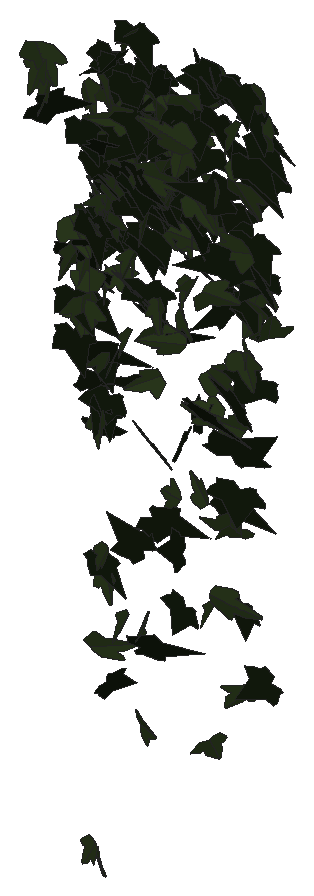
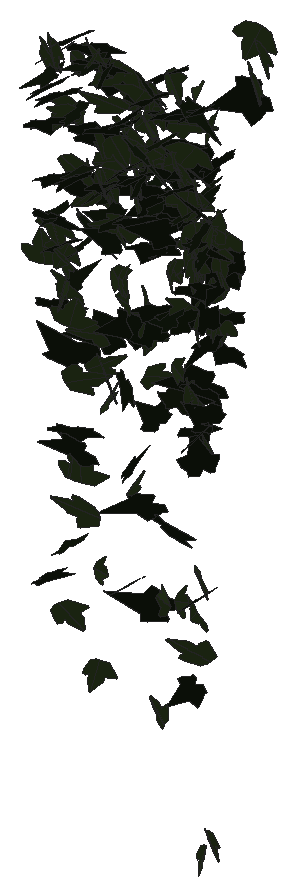
# SketchUp Ruby script. Lengths in millimetres.
U = 1.mm
M = Sketchup.active_model
def pt(a) = Geom::Point3d.new(a.map { |v| v * U })
def face(e, loops, mat)
  f = e.add_face(loops[0].map { |a| pt(a) })
  loops[1..].each { |l| e.add_face(l.map { |a| pt(a) }).erase! }
  f.material = f.back_material = mat if mat
  f
end
# faces: each face lists its corners as indices into pts; further lists are holes
def faces(e, pts, list, mat = nil) = list.each { |f| face(e, (f[0].is_a?(Array) ? f : [f]).map { |l| l.map { |i| pts[i] } }, mat) }
# xy, xz, yz: faces in a plane at the given z, y or x. An outline is a flat list of corners, or four numbers for a rectangle; further outlines are holes
def ring(l) = l.size == 4 ? [[l[0], l[1]], [l[2], l[1]], [l[2], l[3]], [l[0], l[3]]] : l.each_slice(2).to_a
def flat(e, list, mat, &to3) = list.each { |f| face(e, (f[0].is_a?(Array) ? f : [f]).map { |l| ring(l).map { |u, v| to3.(u, v) } }, mat) }
def xy(e, z, list, mat = nil) = flat(e, list, mat) { |x, y| [x, y, z] }
def xz(e, y, list, mat = nil) = flat(e, list, mat) { |x, z| [x, y, z] }
def yz(e, x, list, mat = nil) = flat(e, list, mat) { |y, z| [x, y, z] }
def lines(e, pts, list) = list.each { |a, b| e.add_line(pt(pts[a]), pt(pts[b])) }
# prism: a flat outline (further loops are holes) pulled along v
def prism(e, loops, v, mat = nil)
  f = face(e, loops, mat); d = Geom::Vector3d.new(v.map { |x| x * U })
  f.pushpull(f.normal.samedirection?(d) ? d.length : -d.length)
end
def box(e, o, s, mat = nil) = prism(e, [[o, [o[0] + s[0], o[1], o[2]], [o[0] + s[0], o[1] + s[1], o[2]], [o[0], o[1] + s[1], o[2]]]], [0, 0, s[2]], mat)
def at(x, y, z, deg = 0) = Geom::Transformation.translation(pt([x, y, z])) * Geom::Transformation.rotation(ORIGIN, Z_AXIS, deg.degrees)
def axes(o, x, y, z) = Geom::Transformation.new([*x, 0, *y, 0, *z, 0, *pt(o).to_a, 1])
def part(name) = M.definitions.add(name)
# library, detail: a bought-in or finely detailed component or shape, given as its bounding box
def library(name, o, s) = part(name).tap { |d| box(d.entities, o, s) }
def detail(e, o, s) = box(e.add_group.entities, o, s)
def put(e, d, t, mat = nil) = e.add_instance(d, t).tap { |i| i.material = mat if mat }
def group(e, t, mat = nil) = e.add_group.tap { |g| g.transformation = t; g.material = mat if mat }.entities
root = M.entities
M.materials.add("efeu1").color = [18, 25, 13]
M.materials.add("efeu2").color = [43, 57, 29]
c1 = part("ivyleaf_10")
p = [[0,12.8,-0.8],[-1.5,51.3,-10.9],[-4.9,51,-11.6],[-13.6,26.5,-7.3],[-13.2,15.9,-4.6],[-21.1,19.3,-7.2],
  [-29.5,16.3,-8.3],[-29.2,8.3,-6.2],[-19.7,-9.8,0.5],[-7.6,-13,4],[1,-12.2,5.8],[-0.4,51.1,-11.1],
  [-1.5,51.1,-10.9],[1,-12.4,5.9],[16.9,-12.4,3.5],[35.1,9.1,-5.1],[35,12.9,-6.1],[20.5,16.4,-4.9],
  [15.8,15,-3.8],[15.3,27.6,-7.1],[12.8,31.3,-7.8]]
faces(c1.entities,p,[[0,1,2,3,4,5,6,7,8,9,10],[11,12,0,13,14,15,16,17,18,19,20]],"efeu2")
c2 = part("ivyleaf_9")
p = [[39.1,54.8,31.7],[34.5,51.8,30.2],[-5.3,25.2,17.3],[-17.9,28.3,20.9],[-21.6,21.7,17],[-20.2,4.3,5.3],
  [-22.9,-0.3,2.5],[-17.1,-4,-0.6],[-2,-2.1,-1.2],[-0.7,-15.4,-10.1],[16.6,-22.3,-16.7],[21.1,-15.1,-12.5],
  [32.7,-10.7,-11],[46.1,-1.8,-6.6],[30.8,11.2,3.8]]
faces(c2.entities,p,[[0,1,2,3,4,5,6,7,8,9,10,11,12,13,14]],"efeu1")
put(root,c1,axes([827.3,914.8,1269.9],[-0.03685,-0.91844,-0.1147],[0.01699,0.11429,-0.91888],[1.12908,-0.0317,0.01008]))
put(root,c2,axes([810.5,984.3,656.7],[0.43148,-0.72111,-0.27887],[-0.13514,0.26997,-0.75581],[1.46526,0.23725,0.01241]))
put(root,c1,axes([816.5,990.8,1433.1],[0.58304,-0.45427,0.49056],[0.46498,-0.31033,-0.65866],[0.67017,0.61052,0.03022]))
put(root,c2,axes([814.6,955.2,977],[-0.06259,-0.1793,0.84576],[0.93108,0.38869,0.1287],[-0.49559,0.7529,0.13498]))
put(root,c2,axes([815,917.2,1162.1],[-0.08072,-0.79037,-0.52122],[0.18121,0.50735,-0.7882],[1.14074,-0.13652,0.08832]))
put(root,c1,axes([825.2,950.5,1338.1],[-0.84236,0.60608,-0.07259],[0.08412,-0.03146,-0.91848],[-0.73994,-0.69356,-0.02178]))
put(root,c1,axes([826.2,828.6,1581.8],[0.96241,-0.8078,0.0551],[0.0642,-0.02561,-1.12892],[0.98571,0.79037,0.01973]))
put(root,c2,axes([814.5,970.2,1305.8],[0.80675,-0.56254,-0.10977],[-0.09704,0.07591,-0.86815],[0.69247,0.66601,0.00623]))
put(root,c1,axes([832.2,935.6,168.4],[0.72355,-0.48205,-0.26083],[-0.2237,0.18766,-0.76374],[0.63014,0.62013,0.02837]))
put(root,c1,axes([830.4,897.2,1252.3],[0.06343,-0.81421,0.59742],[0.10119,-0.59274,-0.81506],[1.22788,0.09091,0.03631]))
put(root,c1,axes([828.7,808.1,1627.5],[1.11625,-0.68472,-0.01362],[-0.00812,0.01384,-1.14278],[0.83549,0.91496,0.00709]))
put(root,c1,axes([830.8,966.8,680.9],[0.75004,-0.66968,0.01112],[0.01074,-0.00958,-0.77704],[1.27467,0.39414,0]))
put(root,c2,axes([819.4,971.6,896.5],[1.00535,0.15537,0.12513],[-0.16841,0.06015,0.83438],[0.17571,-0.83133,0.08376]))
put(root,c2,axes([829.7,901.7,1243.4],[0.57474,0.86858,0.16422],[0.0941,0.14499,-0.98811],[-1.07432,0.47737,0.00131]))
put(root,c1,axes([830.9,912.7,1152.6],[-0.32089,-0.95674,0.05571],[0.17709,-0.09687,-0.97836],[1.15571,-0.2508,0.16538]))
put(root,c2,axes([814.6,967.4,1167.5],[-0.16658,-0.25139,0.83172],[0.71275,-0.64976,-0.10048],[0.78464,0.53686,0.26785]))
put(root,c2,axes([832.3,992.7,1245.9],[-0.67217,-0.65377,0.02912],[-0.00914,-0.03177,-0.85484],[0.79834,-0.55081,0.01473]))
put(root,c2,axes([819.6,907.6,1097],[-0.57889,-0.38228,-0.72656],[0.81391,0.30957,-0.59856],[0.58377,-0.81069,0.11404]))
put(root,c1,axes([821.6,984.9,1164.7],[0.39568,-0.50354,0.60933],[0.54283,-0.42808,-0.59059],[0.79708,0.5415,0.09973]))
put(root,c1,axes([815.7,989.8,623.1],[0.90908,-0.34629,0.5412],[0.8315,-0.3194,-0.58998],[0.89659,0.64733,-0.00159]))
put(root,c2,axes([822.2,923.6,1464.6],[0.22176,-0.83835,-0.36779],[-0.07301,0.36329,-0.85766],[1.11449,0.19061,0.017]))
put(root,c2,axes([824.6,945.8,1125.8],[0.31626,-0.49164,-0.71685],[-0.23548,0.69682,-0.5477],[1.03401,0.30907,0.09453]))
put(root,c1,axes([837.8,947.6,142.7],[-0.61671,0.51827,0.32896],[-0.28351,0.23286,-0.72396],[-0.69317,-0.55635,0.00343]))
put(root,c1,axes([836,970.5,1276.3],[-0.1259,-0.84841,-0.28929],[0.02873,0.28853,-0.85459],[1.0932,-0.10529,-0.01086]))
put(root,c2,axes([819.1,976.3,1338.3],[0.5738,-0.73935,0.1343],[0.09718,-0.10849,-0.87622],[0.9116,0.47694,0.00887]))
put(root,c1,axes([825.9,934.6,1157.4],[-0.60213,0.51709,-0.58666],[0.41991,-0.47929,-0.71201],[-0.85669,-0.59837,0.06335]))
put(root,c2,axes([825.7,967.3,1039.2],[-0.48321,-0.46701,-0.61897],[0.59057,0.39403,-0.60704],[0.73897,-0.62027,0.0804]))
put(root,c2,axes([823.1,822.3,1544],[0.04444,0.49674,-1.00223],[0.09991,0.99889,0.49806],[1.361,-0.08955,-0.00384]))
put(root,c2,axes([856.9,952.9,1298.1],[-0.87759,0.06382,0.52703],[-0.64482,-0.00287,-0.72105],[-0.06074,-0.89174,0.04004]))
put(root,c2,axes([832,886.9,1266.4],[1.00556,0.61266,-0.081],[-0.0684,-0.06035,-1.02688],[-0.75084,0.826,-0.01494]))
put(root,c1,axes([834.4,913.6,1239.5],[0.96654,-0.59003,0.14227],[0.15072,-0.07228,-0.9877],[0.72497,0.80166,0.01566]))
put(root,c1,axes([842.5,964.1,1036.4],[-0.28327,-0.87367,0.10082],[-0.03216,-0.09732,-0.90399],[1.07247,-0.23368,-0.00048]))
put(root,c1,axes([834.3,806.9,1651.5],[-1.34063,-0.0535,-0.34198],[0.42219,-0.19472,-1.08151],[-0.00925,-1.13426,0.2018]))
put(root,c2,axes([857.3,961.7,1571.8],[-0.78827,0.67967,-0.20007],[0.06248,-0.21309,-0.79186],[-1.34698,-0.40764,0.08036]))
put(root,c1,axes([833.2,912.9,1143.7],[1.17935,0.20887,0.10557],[0.10249,0.10907,-0.98503],[-0.26649,0.96629,0.08837]))
put(root,c1,axes([839.9,919.6,1187.7],[0.35761,0.91321,-0.25171],[0.08106,0.24301,0.95905],[1.15282,-0.30037,0.01064]))
put(root,c2,axes([840.3,968.3,960.7],[-0.62655,-0.73059,-0.04307],[0.02972,0.03552,-0.89304],[0.89238,-0.51414,-0.0005]))
put(root,c2,axes([831.3,975.3,947.9],[0.11589,-0.86539,0.18702],[0.00654,-0.18752,-0.87047],[1.08013,0.09399,-0.01479]))
put(root,c2,axes([836.2,979.2,1569.9],[-0.28232,-0.79533,0.20841],[0.03217,-0.22358,-0.82392],[1.00254,-0.21679,0.08513]))
put(root,c1,axes([840,962.2,1276.7],[0.2733,-0.74511,0.25395],[0.24362,-0.2326,-0.75486],[1.47825,0.17609,0.07745]))
put(root,c1,axes([839.9,916.4,1534.1],[-0.28327,0.96823,0.01867],[-0.00068,0.01907,-0.99567],[-1.18146,-0.23216,-0.0039]))
put(root,c2,axes([828.3,936.8,1395.7],[0.91204,-0.61799,-0.26415],[-0.31818,0.20461,-0.78199],[1.23889,0.5075,-0.00638]))
put(root,c1,axes([842.3,961.9,1270.2],[0.72661,-0.63739,0.07321],[0.05935,-0.05473,-0.87234],[0.78047,0.59756,-0.00182]))
put(root,c1,axes([838.4,978.7,1497.4],[-1.42032,-0.1447,-0.26511],[0.52164,-0.02761,-0.75648],[0.24146,-0.79149,0.07486]))
put(root,c1,axes([830.1,893.2,1299.6],[1.0073,0.30023,0.54458],[0.63222,0.16817,-0.8784],[-0.41937,0.97468,-0.01619]))
put(root,c2,axes([821.9,951.3,1048.5],[0.23102,0.24737,-0.79483],[0.70014,0.70461,0.27547],[1.4212,-0.38733,-0.00651]))
put(root,c2,axes([833.9,929.7,1410.4],[0.7252,-0.56889,-0.413],[-0.12026,0.46805,-0.78661],[0.84918,0.55212,0.24129]))
put(root,c1,axes([852.8,948.7,1329.2],[-0.61781,-0.73834,0.06604],[-0.0454,-0.05455,-0.89531],[0.90323,-0.50777,0.00017]))
put(root,c1,axes([851,967.8,1040.6],[0.49501,-0.80316,-0.13013],[-0.08958,0.10868,-0.89968],[0.98859,0.41201,-0.01637]))
put(root,c1,axes([846,958.1,1297.8],[0.55063,-0.71531,0.22891],[0.2274,-0.19835,-0.77081],[1.41118,0.31107,0.03489]))
put(root,c2,axes([849.6,955.9,459.9],[-0.04951,0.15388,-0.76833],[-0.50569,0.72148,0.15349],[1.40297,0.26548,0.02821]))
put(root,c1,axes([839.5,943.2,934.3],[0.8773,-0.46081,0.55084],[0.725,-0.39799,-0.65172],[1.15869,0.59792,-0.00928]))
put(root,c2,axes([842,942.7,1283.5],[0.61468,-0.51987,-0.46856],[-0.349,0.43516,-0.60921],[1.28546,0.36674,0.05866]))
put(root,c1,axes([859.3,962.5,1394.7],[-1.26299,-0.42447,-0.01308],[0.0122,0.01425,-0.78771],[0.80813,-0.66359,-0.00855]))
put(root,c2,axes([837,982.5,1380.5],[0.52468,-0.76338,-0.1447],[-0.02366,0.14918,-0.81073],[1.47854,0.27328,0.03838]))
put(root,c2,axes([853.8,976.6,1395.7],[-1.22598,-0.10596,-0.44543],[0.8701,-0.10684,-0.63574],[0.04762,-0.77585,0.14838]))
put(root,c1,axes([835.9,952.8,519.4],[-0.59891,-0.25699,0.66664],[0.96813,0.43092,0.40624],[-0.95481,0.59812,-0.00625]))
put(root,c1,axes([856.6,947.8,1299.5],[-1.06707,0.18745,-0.06691],[0.07914,-0.01663,-0.89451],[-0.22956,-0.87705,0.00266]))
put(root,c1,axes([836.2,901.6,1312],[0.04887,-0.13965,0.93591],[1.14246,-0.12885,-0.0593],[0.166,0.92786,0.13263]))
put(root,c1,axes([853.6,989.7,1468],[1.0977,-0.51262,0.2237],[0.28993,-0.16521,-0.77135],[1.02423,0.59616,-0.0214]))
put(root,c2,axes([859.4,972,1559.8],[-0.51457,-0.76812,0.05811],[-0.03506,-0.05512,-0.81432],[1.46565,-0.271,0.00092]))
put(root,c1,axes([871.5,970.8,1479.7],[-0.08503,-0.79721,-0.08124],[0.02219,0.08071,-0.79843],[1.52495,-0.04563,0.00709]))
put(root,c1,axes([865.6,984.5,1075.2],[0.18999,-0.5844,0.42532],[0.30361,-0.40095,-0.58836],[1.34168,0.17349,0.07291]))
put(root,c1,axes([855.8,968.8,1188.3],[0.7648,0.30394,0.50272],[0.52166,0.26806,-0.69527],[-0.49146,0.75753,0.04432]))
put(root,c1,axes([879.7,938.1,1372.9],[-1.38425,-0.27933,0.11946],[-0.21646,-0.03705,-0.7791],[0.53615,-0.73614,-0.00612]))
put(root,c2,axes([855.3,912.2,1441.4],[1.05483,0.18398,0.3408],[0.39529,0.11309,-0.88305],[-0.25884,0.92245,0.04029]))
put(root,c2,axes([845.6,983.1,1171.1],[0.86645,-0.5011,0.39711],[0.55215,-0.27251,-0.67648],[1.08436,0.53916,0.02715]))
put(root,c1,axes([880.6,978.3,1624.3],[0.02986,-0.83075,0.01138],[-0.05286,-0.0119,-0.83043],[1.58035,0.0153,-0.02799]))
put(root,c2,axes([865.3,975.8,1414.6],[-0.0936,-0.78121,-0.10289],[0.02904,0.10213,-0.78271],[1.49935,-0.05075,0.00874]))
put(root,c2,axes([865.1,899.4,1315.7],[0.17257,-1.01284,0.08061],[0.00573,-0.08074,-1.02265],[1.23956,0.14138,-0.00649]))
put(root,c2,axes([867.3,978.5,1000.3],[-0.43764,-0.81464,0.01399],[0.98174,-0.35663,-0.13333],[0.15569,-0.04108,0.88008]))
put(root,c1,axes([909.1,924.2,1504.4],[0.12914,0.1045,-0.8512],[-1.35399,-0.46995,-0.1144],[-0.91143,0.71295,0.04935]))
put(root,c2,axes([867.1,985.6,1170.9],[0.8548,-0.63915,0.10465],[0.09811,-0.09167,-0.78111],[1.22873,0.45196,-0.01044]))
put(root,c2,axes([917.4,938.3,1449.3],[-0.88049,0.52655,0.39135],[-0.57502,0.25407,-0.69901],[-1.10832,-0.55013,0.05175]))
put(root,c1,axes([878.9,914,1556.1],[-0.14586,-0.23699,0.81822],[1.03542,-0.64577,-0.13608],[1.24752,0.50827,0.20861]))
put(root,c1,axes([886.5,974.1,1241.4],[0.31539,-0.57204,0.53633],[0.64416,-0.4423,-0.57633],[1.3462,0.34566,0.15012]))
put(root,c2,axes([885.5,977.5,1630.9],[0.01718,-0.81708,-0.15844],[0.01211,0.15852,-0.81709],[1.58398,0.00765,0.00797]))
put(root,c1,axes([897.2,953,1242.3],[-0.06309,-0.66304,0.38061],[0.26024,-0.37997,-0.65001],[1.43157,0.03985,0.13494]))
put(root,c1,axes([908.4,926.4,1402],[0.92414,-0.38759,-0.49857],[-0.51187,0.4421,-0.60563],[1.08744,0.53749,0.13862]))
put(root,c2,axes([927.5,941.4,732.5],[-1.28141,0.06996,-0.45742],[-0.86931,0.02883,0.67674],[0.14101,0.81346,0.01535]))
put(root,c1,axes([896.1,937.4,595.6],[0.15187,-0.35651,0.71863],[0.47374,-0.67553,-0.36277],[1.45139,0.2578,0.04321]))
put(root,c2,axes([895.4,960.8,1543.8],[-0.46175,-0.82107,0.00655],[-0.00409,-0.0062,-0.85616],[1.5627,-0.24263,-0.0003]))
put(root,c2,axes([913.7,939,1471.6],[-1.23869,-0.46626,0.07814],[-0.11513,-0.04973,-0.8006],[0.89236,-0.65363,0.00517]))
put(root,c2,axes([889.6,988.8,1501.7],[0.29657,-0.79421,0.00354],[0.00122,-0.00348,-0.80935],[1.51156,0.15583,-0.00004]))
put(root,c2,axes([896.1,962.2,1341.2],[-0.19584,-0.5204,-0.6231],[0.35633,0.59595,-0.52864],[1.50344,-0.20903,0.04412]))
put(root,c2,axes([907.6,982,1175.4],[-0.36294,-0.68504,-0.37729],[0.17046,0.36666,-0.71101],[1.47863,-0.21042,-0.01064]))
put(root,c1,axes([900,977.4,387.5],[-0.46711,0.14957,0.73666],[1.14822,-0.42307,0.2869],[0.85339,0.6511,0.0172]))
put(root,c2,axes([888.7,980.8,1323.7],[1.14436,-0.26249,0.44766],[0.80615,-0.14758,-0.65547],[0.57059,0.73495,0.02826]))
put(root,c1,axes([902.2,941.6,1434.2],[0.7684,-0.34663,0.59315],[1.03453,-0.25955,-0.52168],[0.79959,0.66893,0.10495]))
put(root,c1,axes([935.5,964.9,1028.5],[0.32745,0.19909,-0.76985],[-0.86061,-0.62341,-0.26228],[-1.24485,0.48335,-0.02118]))
put(root,c1,axes([919,959.3,1311.4],[0.60556,-0.66271,0.3683],[0.40536,-0.30521,-0.73318],[1.38485,0.37912,0.05356]))
put(root,c1,axes([928.9,933.2,578],[0.42426,-0.57055,0.53871],[-0.38516,0.49928,0.61253],[-1.4429,-0.30103,-0.00511]))
put(root,c2,axes([908.6,967.8,1367.5],[0.57251,-0.7274,0.2546],[0.16128,-0.24043,-0.78704],[1.45784,0.31225,-0.01291]))
put(root,c1,axes([933.1,967.3,1117.9],[-0.45052,-0.68474,-0.35407],[0.2004,0.33819,-0.72444],[1.45337,-0.25889,-0.00986]))
put(root,c2,axes([901.8,928.3,1408.5],[0.18764,-0.11833,-0.84681],[1.59009,0.19461,0.07008],[0.34607,-0.83002,0.13715]))
put(root,c2,axes([911.2,959.6,1359.8],[-0.36869,-0.19084,-0.77693],[1.07975,0.53085,-0.27185],[1.07354,-0.59946,0.0066]))
put(root,c2,axes([923.3,972.8,1283.1],[-0.54178,-0.66269,-0.37657],[0.30473,0.34101,-0.72116],[1.41827,-0.32642,0.0111]))
put(root,c2,axes([922.6,981.4,1570.9],[-0.13676,-0.82224,-0.03527],[0.01053,0.03492,-0.82537],[1.56629,-0.07203,0.00247]))
put(root,c2,axes([913.1,989.4,1118.9],[0.16574,-0.39271,0.67056],[0.88769,-0.51328,-0.36118],[1.18294,0.4402,0.17708]))
put(root,c2,axes([925.8,952.1,1263.5],[-0.12755,-0.65362,0.40278],[0.27795,-0.40778,-0.63743],[1.43451,0.0209,0.15932]))
put(root,c2,axes([936.9,932.8,1511],[-0.74306,-0.70933,-0.06795],[0.09515,0.05002,-0.80944],[1.35283,-0.39313,0.01961]))
put(root,c1,axes([943.9,960.8,1510.2],[0.50585,-0.7063,0.29734],[0.17142,-0.28374,-0.75451],[1.44838,0.28026,-0.01455]))
put(root,c2,axes([932.9,926.5,1386.7],[-0.25462,-0.65206,0.43289],[0.30937,-0.45274,-0.63173],[1.4571,-0.01782,0.20977]))
put(root,c2,axes([970.5,965.8,1453.9],[-0.83831,0.67683,0.17098],[-0.20886,0.13253,-0.80731],[-1.3121,-0.45353,0.01926]))
put(root,c2,axes([934.2,993.2,1407.7],[0.43695,-0.17133,-0.74563],[1.14548,-0.44014,0.28646],[-0.89889,-0.64417,0.00259]))
put(root,c2,axes([957.8,955.9,1576.1],[-1.1597,0.20437,-0.5192],[0.81946,-0.31675,-0.63001],[-0.67543,-0.73521,0.1271]))
put(root,c2,axes([945.7,991,1335.3],[-0.47467,-0.71427,-0.17879],[0.13356,0.16485,-0.75647],[1.39496,-0.25883,0.01159]))
put(root,c2,axes([952,990.8,1430.8],[-0.71976,-0.65843,0.26314],[0.01495,-0.3021,-0.74463],[1.34942,-0.34785,0.14861]))
put(root,c1,axes([940.3,961.8,1164],[0.85805,-0.40375,0.54214],[0.77291,-0.35917,-0.6052],[1.02844,0.60678,0.00251]))
put(root,c1,axes([955.7,989.8,813.5],[-0.26738,0.48935,0.50558],[0.20018,-0.49516,0.5085],[1.32407,0.17368,0.02522]))
put(root,c1,axes([952.4,929,1514.2],[-1.16331,0.48568,-0.2386],[0.31218,-0.17672,-0.77993],[-0.98141,-0.63191,0.03473]))
put(root,c2,axes([936.3,945.1,931.5],[0.36448,-0.54337,0.58497],[0.42116,-0.54187,-0.57578],[1.45998,0.29196,0.02006]))
put(root,c2,axes([949,990.4,1412.8],[-0.16291,-0.79422,-0.03519],[-0.00387,0.03561,-0.7988],[1.51304,-0.08542,-0.00583]))
put(root,c2,axes([938.6,962.5,781.4],[0.42736,-0.07733,-0.8202],[0.22047,0.84464,-0.04792],[1.55235,-0.09867,0.23261]))
put(root,c1,axes([973.2,927.5,1548.6],[-1.17822,0.40829,0.35636],[-0.5646,0.19745,-0.74158],[-0.86315,-0.68648,-0.00136]))
put(root,c1,axes([969.1,948.3,1434],[-0.38395,-0.81669,0.01919],[-0.00556,-0.01905,-0.84123],[1.55474,-0.20175,0.00173]))
put(root,c1,axes([981,957.7,1112.2],[0.061,0.08121,0.82664],[-0.68266,-0.74479,0.08707],[1.42583,-0.36007,0.00632]))
put(root,c2,axes([945,970.1,1392.2],[-0.14928,-0.31986,-0.74528],[0.83169,0.6141,-0.30955],[1.3003,-0.42951,0.11243]))
put(root,c1,axes([971.1,958.1,1375.5],[-0.06928,-0.81137,-0.1848],[0.06748,0.1833,-0.81175],[1.58231,-0.04334,0.02652]))
put(root,c2,axes([939,932.1,563.6],[0.61971,-0.01227,0.75109],[1.42891,0.0319,-0.32496],[-0.04642,0.81801,0.02394]))
put(root,c1,axes([978.5,951.2,1399.4],[0.43289,-0.63084,-0.51206],[-0.25157,0.49593,-0.66969],[1.52576,0.26075,0.03486]))
put(root,c2,axes([986.6,984.3,1502.8],[-0.62613,-0.68329,0.30857],[0.23752,0.28235,0.75831],[-1.40699,0.35174,-0.0093]))
put(root,c2,axes([975.5,947.6,1499],[-0.60959,-0.7039,0.37229],[-0.31978,-0.3325,-0.77323],[1.48138,-0.36143,-0.01372]))
put(root,c2,axes([972.3,992.9,620.2],[-0.36378,-0.61525,0.418],[-0.20113,-0.40474,-0.64406],[1.40126,-0.21782,0.01607]))
put(root,c2,axes([962.5,975.4,1427.8],[0.5553,-0.60977,-0.41938],[-0.17491,0.41745,-0.6709],[1.39759,0.29452,0.08266]))
put(root,c2,axes([966.5,961.8,1111.8],[-0.03415,0.43454,-0.70073],[-0.0144,0.70078,0.43477],[1.56919,0.01589,-0.01126]))
put(root,c1,axes([959.7,952.3,1497.6],[0.9628,-0.31608,0.5704],[0.94265,-0.28337,-0.5963],[0.80734,0.7078,0.016]))
put(root,c1,axes([969.3,945.1,1547.6],[1.36056,0.32118,0.26593],[0.42654,0.14913,-0.7826],[-0.66924,0.74802,0.04184]))
put(root,c2,axes([986.8,936.9,1514.9],[0.62803,-0.24303,-0.74984],[-1.08912,0.48517,-0.40908],[1.03169,0.66013,0.0246]))
put(root,c2,axes([991.4,904.9,1517.3],[-0.54686,0.68274,-0.50501],[-0.49269,0.43734,0.73855],[1.53931,0.38254,0.05698]))
put(root,c1,axes([991.7,985.7,1210.9],[0.02542,-0.78462,0.19416],[0.0799,-0.19325,-0.78383],[1.53625,0.02304,0.03756]))
put(root,c1,axes([957.8,919.9,1419.5],[-0.2359,-0.06632,0.87594],[1.62493,0.19901,0.13588],[-0.3933,0.86199,0.03602]))
put(root,c1,axes([981.2,985.4,1205.9],[0.11973,-0.49702,0.63173],[0.62404,-0.56268,-0.47535],[1.39676,0.294,0.15822]))
put(root,c1,axes([999.7,981,1457.1],[-0.53038,-0.71802,0.24819],[-0.11271,-0.24303,-0.76957],[1.44147,-0.28319,0.03115]))
put(root,c1,axes([980.1,972.6,1156.4],[0.3009,-0.24491,0.75063],[1.14513,-0.45833,-0.27627],[0.97306,0.61512,0.09301]))
put(root,c1,axes([989.2,981.2,1292.2],[0.59138,-0.37169,0.60793],[0.84661,-0.41692,-0.48227],[1.05941,0.54066,0.04604]))
put(root,c1,axes([980.2,969,1302.3],[-0.51325,-0.17728,-0.76835],[1.43762,0.17496,-0.30549],[0.43068,-0.79529,0.10407]))
put(root,c1,axes([1037.7,901.6,1516.2],[0.63285,0.07041,0.85628],[-1.5834,-0.20282,0.33976],[0.40819,-0.89591,-0.00962]))
put(root,c1,axes([1005.1,943.5,1469.4],[1.35775,-0.44841,0.12117],[0.17973,-0.07741,-0.84249],[0.86556,0.71947,-0.01513]))
put(root,c2,axes([1028.2,917.7,962.7],[-0.38655,0.20716,-0.8038],[-1.12391,0.54547,0.2898],[1.11019,0.62434,0.01351]))
put(root,c2,axes([1006.6,978.7,974.3],[-0.03219,0.46499,0.67833],[0.01021,-0.67839,0.46517],[1.56516,0.01399,0.01092]))
put(root,c1,axes([1026.9,967,1380.2],[1.1549,-0.18759,-0.47779],[-0.48533,0.53188,-0.5327],[0.84782,0.56001,0.3459]))
put(root,c2,axes([1030.4,977.4,1570.3],[-0.19191,-0.50517,0.65479],[0.26058,0.64033,0.5151],[-1.55224,0.16995,0.00552]))
put(root,c2,axes([1018.3,976.9,1369.4],[-0.62393,-0.70465,-0.13201],[0.07987,0.12605,-0.77703],[1.36208,-0.33017,-0.01491]))
put(root,c2,axes([1001.8,979.6,1310.1],[0.69116,-0.6093,0.3279],[0.36035,-0.26868,-0.70895],[1.26662,0.40892,0.02277]))
put(root,c1,axes([1023.6,994.8,637.9],[0.18782,-0.42814,0.5521],[0.32859,-0.52534,-0.43825],[1.28843,0.19639,0.03129]))
put(root,c2,axes([999.6,970.7,1263.2],[0.77104,-0.55256,0.4427],[0.56086,-0.33217,-0.68429],[1.22525,0.49977,0.03465]))
put(root,c2,axes([1035.3,904.4,778.8],[-0.20133,-0.06323,0.8525],[-0.75003,-0.75867,-0.10517],[1.44374,-0.40295,0.06425]))
put(root,c2,axes([1035.8,973.7,1470.2],[-0.81634,-0.65321,0.1995],[-0.14495,-0.18837,-0.7805],[1.29178,-0.43394,0.03849]))
put(root,c1,axes([1035.3,972.1,1368.9],[0.48339,-0.74426,0.11013],[0.09197,-0.09986,-0.78629],[1.42893,0.2582,0.01335]))
put(root,c2,axes([1025.4,993.8,1355.1],[-0.06916,-0.73191,0.28257],[-0.06528,-0.28112,-0.73257],[1.49175,-0.04624,-0.01896]))
put(root,c1,axes([1027.1,937.2,1571.6],[-1.3558,-0.24353,-0.44707],[0.79058,0.16647,-0.75259],[0.56015,-0.8244,-0.01991]))
put(root,c1,axes([1049.5,967.7,1004.6],[0.15316,0.45646,0.69902],[-0.35922,-0.67413,0.46193],[1.54776,-0.20163,0.03804]))
put(root,c2,axes([1025.3,956.2,1338.6],[0.10898,-0.69106,0.4869],[0.06079,-0.4859,-0.69339],[1.60774,0.06522,-0.00679]))
put(root,c2,axes([1032.8,934.4,1547.8],[-0.5287,-0.76858,-0.28687],[0.15768,0.27503,-0.81711],[1.55335,-0.28952,-0.01469]))
put(root,c1,axes([1015.9,955.7,1511.7],[0.76581,-0.04089,-0.73721],[1.33681,0.27994,0.36786],[0.43306,-0.79184,0.16811]))
put(root,c2,axes([1048.3,975.1,1591.1],[-1.29498,-0.47929,-0.10624],[0.31791,-0.05529,-0.82038],[0.87858,-0.68644,0.14026]))
put(root,c1,axes([1048.5,972.2,1609.6],[-0.28716,0.81193,-0.1575],[0.0525,-0.15507,-0.82583],[-1.5732,-0.15338,0.00119]))
put(root,c1,axes([1078.5,990.1,979.8],[-0.52801,-0.1483,-0.76142],[-1.30137,-0.33514,0.31442],[-0.69722,0.73785,-0.01023]))
put(root,c1,axes([1054.7,956,424.3],[-0.57182,-0.6959,-0.35345],[0.32383,0.31122,-0.7574],[1.44975,-0.344,0.02977]))
put(root,c1,axes([1054,972.5,1615.5],[1.08513,-0.61617,0.07402],[0.09415,-0.05507,-0.83949],[1.17737,0.5723,-0.00108]))
put(root,c2,axes([1064.5,969.5,1615.9],[-1.13784,-0.59185,-0.04026],[0.04894,0.03126,-0.84125],[1.12795,-0.59839,-0.00412]))
put(root,c1,axes([1036.7,938.6,1391.8],[1.04001,-0.12403,0.64479],[1.19716,-0.14169,-0.56035],[0.35838,0.83324,0.00069]))
put(root,c2,axes([1044.9,974.8,1595.7],[0.87665,-0.69476,-0.084],[0.05615,0.11975,-0.82867],[1.33071,0.45264,0.0903]))
put(root,c1,axes([1069.6,983.6,797.4],[-1.50169,-0.20927,0.0502],[0.1307,-0.06404,0.81244],[-0.38816,0.78803,0.07936]))
put(root,c1,axes([1076.4,935.5,1434.8],[0.82837,-0.59326,-0.33798],[-0.1957,0.33929,-0.72797],[1.28465,0.43423,0.10704]))
put(root,c2,axes([1102.8,938,1419.7],[-0.67905,-0.02374,0.79988],[-1.4894,-0.17258,-0.3542],[0.31812,-0.85867,0.04907]))
put(root,c1,axes([1080.2,902.7,894.8],[-0.42066,0.84584,0.06133],[-0.01788,-0.06582,0.87387],[1.61394,0.21973,0.02567]))
put(root,c2,axes([1070.9,989.8,1379.4],[-0.45202,-0.66097,0.36817],[0.06499,-0.39486,-0.68685],[1.43848,-0.18986,0.14672]))
put(root,c1,axes([1050.5,966.3,1068.7],[0.75462,-0.01317,0.74077],[1.41005,0.00762,-0.39643],[-0.00096,0.84017,0.01521]))
put(root,c1,axes([1090.1,985.8,1089.3],[-1.19484,-0.39783,-0.1863],[-0.30382,-0.09612,0.74323],[-0.77889,0.64777,-0.00412]))
put(root,c2,axes([1055.2,912.8,1042.1],[1.48396,-0.36529,0.31679],[0.53519,-0.14641,-0.86095],[0.7486,0.82878,-0.01247]))
put(root,c1,axes([1070.6,959,1359.9],[0.64155,-0.49446,0.61025],[0.9442,-0.38078,-0.58258],[1.15886,0.58398,0.13683]))
put(root,c1,axes([1089,963,819.2],[-0.40598,-0.53067,-0.48237],[0.29887,0.45648,-0.57163],[1.33173,-0.26422,-0.01877]))
put(root,c2,axes([1078.2,986.1,1368],[0.11982,-0.73518,-0.27479],[-0.02046,0.27484,-0.73777],[1.4936,0.06275,0.01194]))
put(root,c2,axes([1075.4,973.6,1229.8],[0.54942,-0.7047,-0.12037],[-0.05916,0.11731,-0.76138],[1.35933,0.28994,0.01551]))
put(root,c2,axes([1076.3,982.5,1489.8],[0.75991,-0.70619,-0.07102],[-0.03277,0.07183,-0.811],[1.3504,0.39914,0.02029]))
put(root,c2,axes([1066.3,984.2,847.6],[0.24882,-0.17181,-0.73096],[1.24612,0.38931,0.0256],[0.6996,-0.63233,0.21437]))
put(root,c2,axes([1084.8,996.6,661.6],[-0.09466,-0.72483,0.33388],[0.02308,-0.33518,-0.72584],[1.51864,-0.04009,0.03184]))
put(root,c2,axes([1092.9,979.4,877.2],[-0.90694,-0.55415,-0.24516],[0.29868,0.18839,-0.73086],[1.11392,-0.5017,-0.00364]))
put(root,c1,axes([1110.7,977.2,524.8],[-0.66383,-0.56177,0.39572],[-0.39903,-0.33561,-0.66124],[1.24542,-0.40696,-0.00094]))
put(root,c2,axes([1084.4,938,1559.5],[0.11309,-0.80729,0.18536],[0.04977,-0.18392,-0.80938],[1.57562,0.06375,0.01226]))
put(root,c2,axes([1124.5,928.3,1318.9],[-0.25128,-0.2864,-0.82409],[-0.49377,-0.78287,0.31364],[-1.5853,0.28924,0.03293]))
put(root,c2,axes([1120.9,914.1,1240],[-1.23416,0.55639,-0.23985],[0.33522,-0.16303,-0.8544],[-1.10333,-0.6719,0.0087]))
put(root,c1,axes([1107.6,979.3,1217.3],[-1.33517,0.2744,-0.0475],[0.0992,0.00292,-0.75298],[-0.52063,-0.70314,-0.02167]))
put(root,c1,axes([1116.6,966.3,1132.9],[0.42541,-0.47181,-0.62714],[0.12879,0.66124,-0.47335],[1.48807,0.07766,0.22025]))
put(root,c1,axes([1107,962.1,1473.2],[0.64918,0.60844,0.42613],[0.24228,0.41409,-0.69315],[-1.39282,0.35562,0.07804]))
put(root,c1,axes([1141,924.4,1346.3],[0.76967,-0.28145,-0.72665],[-1.1717,0.38649,-0.49233],[0.90919,0.73634,-0.01933]))
put(root,c2,axes([1108.6,960.5,1612.4],[-0.13876,-0.83658,0.02971],[0.00136,-0.02989,-0.83975],[1.59319,-0.07284,0.0033]))
put(root,c1,axes([1088.5,940.1,699.3],[-0.10477,0.03823,-0.87724],[1.55306,-0.32231,-0.06525],[-0.61704,-0.81774,-0.01529]))
put(root,c1,axes([1121.5,978.8,1202.6],[1.15787,-0.5967,0.00898],[0.01289,-0.00591,-0.85216],[1.1357,0.60842,0.00052]))
put(root,c2,axes([1131.9,988.3,1275.3],[-1.38062,-0.17452,-0.17811],[0.32868,0.04363,-0.74611],[0.34234,-0.74569,-0.00197]))
put(root,c2,axes([1115.5,981,1222.6],[-0.16433,-0.75429,-0.01122],[-0.00555,0.01162,-0.7592],[1.43571,-0.08629,-0.00422]))
put(root,c1,axes([1115.1,875.4,1284.9],[-0.54616,-0.47046,-0.793],[0.88349,0.64387,-0.54998],[1.51624,-0.54464,0.03482]))
put(root,c1,axes([1124.1,930.6,1557.9],[0.22234,-0.66008,0.56389],[0.39916,-0.53066,-0.66464],[1.60332,0.22365,0.08727]))
put(root,c2,axes([1143.1,966.8,1097.6],[-1.26898,-0.40237,0.01917],[-0.03091,-0.01018,-0.77877],[0.76604,-0.66696,0.00032]))
put(root,c1,axes([1134.5,974.7,1253],[1.38856,-0.17745,-0.13262],[-0.15971,0.20108,-0.73069],[0.3902,0.71377,0.17287]))
put(root,c1,axes([1116.1,956.9,1129.5],[1.24175,-0.25281,0.5036],[0.89937,-0.17419,-0.69969],[0.58416,0.80558,0.00674]))
put(root,c1,axes([1135.6,977,1600],[0.99361,-0.6319,-0.15656],[0.0654,0.22715,-0.80224],[1.23728,0.49545,0.16813]))
put(root,c2,axes([1121.2,984.2,1279.5],[0.39311,-0.75847,0.16522],[0.07444,-0.16058,-0.78608],[1.4755,0.21018,-0.00436]))
put(root,c2,axes([1138.7,991.7,1456.1],[-0.70215,-0.71035,-0.07434],[0.05407,0.06901,-0.80041],[1.35824,-0.36997,-0.00657]))
put(root,c2,axes([1129.9,965.3,1344.7],[-0.19049,-0.79739,-0.26224],[0.17761,0.25189,-0.80153],[1.58765,-0.12385,0.0582]))
put(root,c2,axes([1123.6,925.9,975.6],[-0.56488,-0.10776,0.86627],[1.63136,-0.20915,0.26767],[0.31444,0.8915,0.16751]))
put(root,c2,axes([1130.1,971.6,1458.8],[0.42559,-0.74609,-0.22897],[0.00728,0.23923,-0.77579],[1.48531,0.21261,0.06941]))
put(root,c1,axes([1139.4,926.7,1457.1],[-1.39248,0.39673,-0.31358],[0.50675,-0.16665,-0.83209],[-0.81823,-0.77838,0.01832]))
put(root,c2,axes([1131.2,979.5,1545.2],[0.94629,-0.61826,-0.23493],[-0.14827,0.23712,-0.7889],[1.25,0.49617,0.08428]))
put(root,c2,axes([1137.8,977,1520.7],[0.33389,-0.74114,-0.30585],[-0.06536,0.30586,-0.76084],[1.52453,0.17543,0.03437]))
put(root,c2,axes([1136.4,953.2,1494.3],[0.16301,-0.79889,-0.33388],[0.11108,0.34007,-0.79874],[1.64415,0.05623,0.08706]))
put(root,c2,axes([1142.3,963.8,1573.2],[-0.02167,-0.817,0.15386],[-0.05384,-0.1534,-0.81668],[1.58134,-0.01642,-0.0257]))
put(root,c2,axes([1163.4,967.3,560.9],[-0.67592,-0.43073,0.55439],[-0.61309,-0.45204,-0.55758],[1.18718,-0.47868,0.0277]))
put(root,c1,axes([1183,941.9,1557.4],[-0.03661,0.16408,0.83402],[-1.37407,0.43714,-0.10265],[-0.85381,-0.71054,0.12944]))
put(root,c2,axes([1170.6,889.3,1084.3],[0.25485,-0.85102,0.27522],[-0.0817,0.27185,0.86149],[-1.70029,-0.14062,-0.00014]))
put(root,c1,axes([1160.1,973.7,1182.6],[-0.71273,-0.75009,-0.1809],[-0.09192,-0.17789,0.83762],[-1.46561,0.37592,0.03543]))
